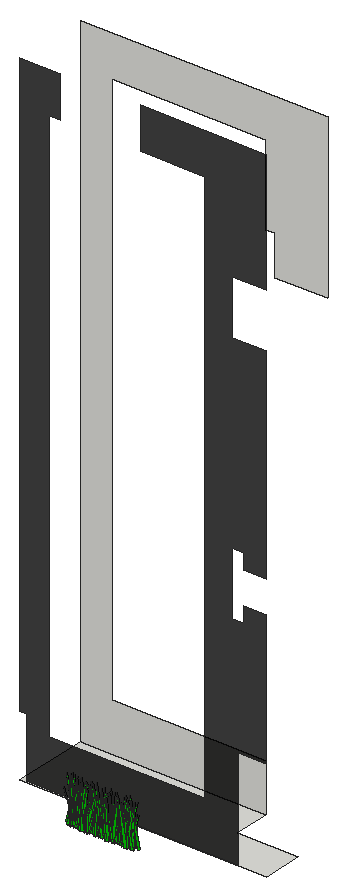
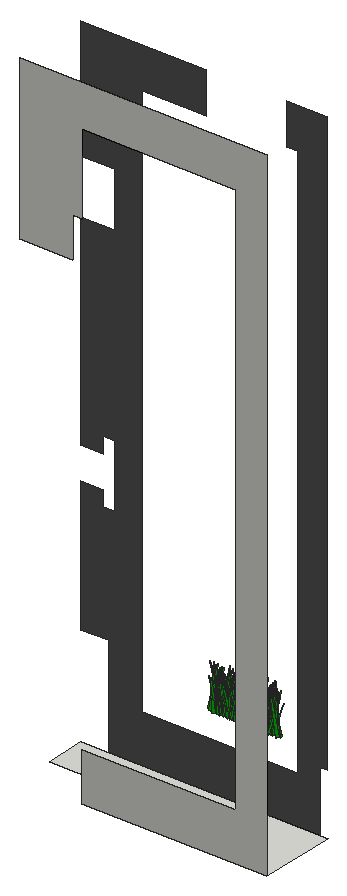
# SketchUp Ruby script. Lengths in inches.
U = 1.inch
M = Sketchup.active_model
def pt(a) = Geom::Point3d.new(a.map { |v| v * U })
def face(e, loops, mat)
  f = e.add_face(loops[0].map { |a| pt(a) })
  loops[1..].each { |l| e.add_face(l.map { |a| pt(a) }).erase! }
  f.material = f.back_material = mat if mat
  f
end
# faces: each face lists its corners as indices into pts; further lists are holes
def faces(e, pts, list, mat = nil) = list.each { |f| face(e, (f[0].is_a?(Array) ? f : [f]).map { |l| l.map { |i| pts[i] } }, mat) }
# xy, xz, yz: faces in a plane at the given z, y or x. An outline is a flat list of corners, or four numbers for a rectangle; further outlines are holes
def ring(l) = l.size == 4 ? [[l[0], l[1]], [l[2], l[1]], [l[2], l[3]], [l[0], l[3]]] : l.each_slice(2).to_a
def flat(e, list, mat, &to3) = list.each { |f| face(e, (f[0].is_a?(Array) ? f : [f]).map { |l| ring(l).map { |u, v| to3.(u, v) } }, mat) }
def xy(e, z, list, mat = nil) = flat(e, list, mat) { |x, y| [x, y, z] }
def xz(e, y, list, mat = nil) = flat(e, list, mat) { |x, z| [x, y, z] }
def yz(e, x, list, mat = nil) = flat(e, list, mat) { |y, z| [x, y, z] }
def lines(e, pts, list) = list.each { |a, b| e.add_line(pt(pts[a]), pt(pts[b])) }
# prism: a flat outline (further loops are holes) pulled along v
def prism(e, loops, v, mat = nil)
  f = face(e, loops, mat); d = Geom::Vector3d.new(v.map { |x| x * U })
  f.pushpull(f.normal.samedirection?(d) ? d.length : -d.length)
end
def box(e, o, s, mat = nil) = prism(e, [[o, [o[0] + s[0], o[1], o[2]], [o[0] + s[0], o[1] + s[1], o[2]], [o[0], o[1] + s[1], o[2]]]], [0, 0, s[2]], mat)
def at(x, y, z, deg = 0) = Geom::Transformation.translation(pt([x, y, z])) * Geom::Transformation.rotation(ORIGIN, Z_AXIS, deg.degrees)
def axes(o, x, y, z) = Geom::Transformation.new([*x, 0, *y, 0, *z, 0, *pt(o).to_a, 1])
def part(name) = M.definitions.add(name)
# library, detail: a bought-in or finely detailed component or shape, given as its bounding box
def library(name, o, s) = part(name).tap { |d| box(d.entities, o, s) }
def detail(e, o, s) = box(e.add_group.entities, o, s)
def put(e, d, t, mat = nil) = e.add_instance(d, t).tap { |i| i.material = mat if mat }
def group(e, t, mat = nil) = e.add_group.tap { |g| g.transformation = t; g.material = mat if mat }.entities
root = M.entities
M.materials.add("[Color G06]").color = [0, 204, 0]
M.materials.add("[Color I07]").color = [0, 0, 0]
M.materials["[Color I07]"].alpha = 0.79
c1 = part("fur_instance\#9")
p = [[0.8125,0,1.79],[0.67,-0.02,1.48],[0,-0.11,0],[0,0.11,0]]
faces(c1.entities,p,[[0,1,2,3]])
xy(root,-6,[[0,50.4375,0,79.8125,71,79.8125,71,65.625,94.55,65.625,94.55,50.4375]])
xz(root,50.4375,[[2.44,-6,84.05,-6,84.05,32.52,94.55,32.52,94.55,84,85.8,84.0625,85.8,78.0625,81.61,78.0625,81.61,102,85.8,102,85.8,96,94.55,96,94.55,174.6875,81.61,174.6875,81.61,195.375,94.55,195.375,94.55,242.375,46.35,242.375,46.35,226.18,71,226.18,71,12.68,11.58,12.68,11.58,226.18,15.47,226.18,15.47,242.375,0,242.375,0,17.375,2.44,17.375]],"[Color I07]")
xz(root,79.8125,[[0,-6,0,242.375,94.55,242.375,94.55,180,74.48,180,74.48,195.375,71,195.375,71,226.18,11.58,226.18,11.58,12.68,71,12.68,71,-6]])
put(root,c1,axes([44.51,23.2,4.28],[-3.54509,0.14274,0.85151],[0.77212,0.47511,-1.96873],[0.88106,0.15798,5.15148]),"[Color G06]")
put(root,c1,axes([45.09,23.48,4.28],[-1.82166,0.34556,1.78414],[2.70884,0.19069,1.93525],[-0.4778,-0.23637,4.16953]),"[Color G06]")
put(root,c1,axes([46.25,23.55,4.28],[-4.84362,0.37826,3.53182],[3.333,0.67983,1.8462],[1.3541,-0.32032,8.08908]),"[Color G06]")
put(root,c1,axes([43.88,23.57,4.28],[-3.95994,-0.13546,0.88932],[-0.84613,0.5507,1.22032],[0.76279,-0.09238,5.97047]),"[Color G06]")
put(root,c1,axes([49.65,23.55,4.28],[5.17923,0.26142,3.18644],[2.36605,-0.73928,-1.62302],[-1.56903,-0.25188,8.07066]),"[Color G06]")
put(root,c1,axes([50.67,23.32,4.28],[-2.69769,0.27399,1.06941],[1.83268,0.38822,-1.0992],[1.007,0.02748,4.86538]),"[Color G06]")
put(root,c1,axes([56.88,23.5625,4.28],[-4.25805,0.04028,1.29058],[0.46192,0.59179,1.28248],[0.78468,-0.12979,6.24834]),"[Color G06]")
put(root,c1,axes([45.7,23.27,4.28],[2.11895,0.70671,1.8047],[4.98939,-0.32759,1.65079],[-1.49964,-0.09135,8.04226]),"[Color G06]")
put(root,c1,axes([62.1,23.4375,4.28],[-1.88004,0.75275,2.43709],[5.58061,0.21393,2.02573],[-0.81003,-0.27325,8.29964]),"[Color G06]")
put(root,c1,axes([51.63,23.65,4.28],[4.44552,0.10549,2.58087],[1.22575,-0.63033,-1.75656],[-1.43239,-0.21201,6.50674]),"[Color G06]")
put(root,c1,axes([60.68,23.37,4.28],[-4.22727,-0.07602,1.84569],[-0.86752,0.5867,-1.66245],[1.03423,0.18142,6.14953]),"[Color G06]")
put(root,c1,axes([56.74,23.71,4.28],[-0.19459,-0.67981,1.29759],[-4.77626,0.05774,1.87526],[1.30687,0.10981,7.04678]),"[Color G06]")
put(root,c1,axes([46.61,23.25,4.28],[-6.08695,0.08552,0.82543],[0.38611,0.80168,-3.18156],[0.72944,0.28931,8.57207]),"[Color G06]")
put(root,c1,axes([40.97,23.76,4.28],[5.65286,-0.0501,2.42135],[0.07547,-0.79345,-2.27951],[-1.65774,-0.20696,8.15299]),"[Color G06]")
put(root,c1,axes([45.35,23.61,4.28],[4.08445,-0.33976,0.05652],[-2.40368,-0.56006,1.2612],[0.40036,0.10372,6.99537]),"[Color G06]")
put(root,c1,axes([54.27,23.35,4.28],[2.99814,0.33718,1.93611],[1.78076,-0.44278,2.69852],[-2.08657,0.1066,5.08498]),"[Color G06]")
put(root,c1,axes([62.9,23.31,4.28],[2.88924,0.4246,0.75633],[2.60876,-0.38757,2.7335],[-1.64986,0.13074,5.64669]),"[Color G06]")
put(root,c1,axes([54.14,23.91,4.28],[3.12472,-0.62007,0.24573],[-4.34541,-0.43125,-1.5795],[-0.9578,-0.06637,7.96762]),"[Color G06]")
put(root,c1,axes([47.5,23.3125,4.28],[-3.39734,0.42812,0.33611],[2.84215,0.45416,-2.28278],[1.1826,0.13839,6.45178]),"[Color G06]")
put(root,c1,axes([62.16,23.56,4.28],[1.75413,0.72883,2.24788],[5.36188,-0.19484,-2.08953],[0.91096,-0.25663,7.97043]),"[Color G06]")
put(root,c1,axes([44.98,23.57,4.28],[2.73301,-0.63153,3.24486],[-5.02072,-0.33463,1.96447],[0.12991,0.35344,7.65778]),"[Color G06]")
put(root,c1,axes([47.04,23.35,4.28],[-3.80873,0.3681,0.6701],[2.34921,0.51156,-2.45531],[1.28475,0.15586,6.47617]),"[Color G06]")
put(root,c1,axes([43.07,23.8,4.28],[1.98494,-0.79883,1.68409],[-5.72424,-0.23362,2.34093],[1.14892,0.21616,8.75366]),"[Color G06]")
put(root,c1,axes([45.58,23.59,4.28],[-1.2576,0.4007,0.15915],[2.65614,0.15567,1.86003],[-1.10158,-0.08211,4.30322]),"[Color G06]")
put(root,c1,axes([52.92,23.53,4.28],[-1.37532,0.6451,0.86713],[4.61456,0.17628,1.28324],[-0.66623,-0.11068,7.09816]),"[Color G06]")
put(root,c1,axes([55.78,23.5,4.28],[-4.40695,-0.23643,2.93875],[-2.38236,0.58297,-2.59258],[1.03211,0.33612,6.56368]),"[Color G06]")
put(root,c1,axes([55.19,23.55,4.28],[0.9786,0.78748,2.4969],[5.61272,-0.19622,2.19507],[-1.78308,-0.18545,8.27993]),"[Color G06]")
put(root,c1,axes([64.37,23.54,4.28],[-0.38469,0.60361,0.86334],[4.16993,0.02675,2.00178],[-1.2972,-0.09301,6.17884]),"[Color G06]")
put(root,c1,axes([41.99,23.87,4.28],[-3.48804,-0.11817,2.16828],[-0.42937,0.51339,1.67127],[1.62435,-0.11805,5.09781]),"[Color G06]")
put(root,c1,axes([52.0625,23.68,4.28],[2.23393,0.42821,3.02957],[3.13811,-0.39438,1.23473],[-1.9212,-0.14628,5.53956]),"[Color G06]")
put(root,c1,axes([55.55,24.03,4.28],[2.10305,-0.67058,1.59322],[-4.42122,-0.32824,-2.83456],[-2.17141,0.01886,7.31451]),"[Color G06]")
put(root,c1,axes([48.33,23.55,4.28],[5.20728,0.24689,0.32404],[1.69027,-0.71279,1.71182],[-0.56976,0.14181,8.03999]),"[Color G06]")
put(root,c1,axes([57.11,24.25,4.28],[-5.38239,-0.42009,0.46162],[-2.5521,0.6765,4.25161],[1.63026,-0.32792,8.17975]),"[Color G06]")
put(root,c1,axes([61.32,23.51,4.28],[-0.30876,0.76243,0.46443],[5.41529,0.04897,-1.19389],[0.81616,-0.03651,8.09724]),"[Color G06]")
put(root,c1,axes([46.4375,23.64,4.28],[3.12548,0.67267,0.38577],[4.72579,-0.41686,-2.02486],[1.00176,-0.13219,8.34865]),"[Color G06]")
put(root,c1,axes([56.5,23.95,4.28],[4.12533,0.2555,0.67281],[1.83219,-0.50648,-3],[0.4503,-0.2799,6.04264]),"[Color G06]")
put(root,c1,axes([46.74,23.92,4.28],[-3.06003,-0.07059,0.14472],[-0.46957,0.41537,1.09426],[0.21238,-0.09863,4.50459]),"[Color G06]")
put(root,c1,axes([55.53,24.21,4.28],[6.01483,-0.23374,0.31839],[-1.46727,-0.77699,-3.60972],[-0.83799,-0.31726,8.60576]),"[Color G06]")
put(root,c1,axes([39.93,23.67,4.28],[2.75325,0.66588,0.22772],[4.68443,-0.37143,-1.74762],[0.939,-0.09946,8.05067]),"[Color G06]")
put(root,c1,axes([47.41,23.89,4.28],[2.57672,-0.41829,1.05478],[-3.02777,-0.31979,1.95383],[0.57331,0.19112,5.57789]),"[Color G06]")
put(root,c1,axes([63.42,24.03,4.28],[4.38595,0.08594,2.1676],[0.96165,-0.6198,-1.52342],[-1.24839,-0.1755,6.44184]),"[Color G06]")
put(root,c1,axes([54.99,24.08,4.28],[-1.28026,-0.58457,0.66085],[-4.17293,0.16664,-1.1253],[-0.59651,0.08891,6.45369]),"[Color G06]")
put(root,c1,axes([64.34,23.76,4.28],[-2.6052,0.64918,1.97946],[4.64475,0.39431,-1.20009],[1.36139,-0.10299,7.88241]),"[Color G06]")
put(root,c1,axes([61.91,23.91,4.28],[2.69159,0.31638,0.03082],[2.17504,-0.35851,-1.53288],[0.64596,-0.11113,5.03305]),"[Color G06]")
put(root,c1,axes([40.33,24.14,4.28],[5.72745,-0.10287,2.95356],[-0.26545,-0.82618,-2.1557],[-2.09263,-0.17675,8.35726]),"[Color G06]")
put(root,c1,axes([49.69,24.2,4.28],[1.41781,-0.56666,0.72438],[-3.7532,-0.20856,-2.33225],[-1.63149,-0.01267,5.9948]),"[Color G06]")
put(root,c1,axes([41.3125,24,4.28],[3.06688,-0.45258,0.09249],[-3.0522,-0.39799,2.35446],[1.10535,0.15676,6.24473]),"[Color G06]")
put(root,c1,axes([42.89,23.9,4.28],[2.5172,0.59368,1.6217],[4.37953,-0.32514,-1.51125],[0.35053,-0.20096,7.23591]),"[Color G06]")
put(root,c1,axes([61.48,24.17,4.28],[3.38185,-0.03705,1.52445],[0.18095,-0.4505,-2.15437],[-1.03838,-0.19917,4.58951]),"[Color G06]")
put(root,c1,axes([42.625,24.0625,4.28],[-4.9972,0.13364,2.38193],[1.22394,0.71608,1.1205],[1.40014,-0.14899,7.52179]),"[Color G06]")
put(root,c1,axes([63.49,24.09,4.28],[-2.77989,0.07928,2.11152],[0.98461,0.40638,1.14286],[1.16178,-0.15471,4.08385]),"[Color G06]")
put(root,c1,axes([48.11,24.16,4.28],[3.30766,-0.41695,1.64743],[-2.87103,-0.48603,-1.25458],[-1.38293,0.01178,6.54484]),"[Color G06]")
put(root,c1,axes([61.75,24.06,4.28],[-2.77391,0.20467,0.40541],[1.46966,0.36059,1.55019],[-0.26061,-0.14501,4.42682]),"[Color G06]")
put(root,c1,axes([44.8,24.05,4.28],[1.74896,-0.40041,0.88785],[-2.85294,-0.21008,1.66982],[0.67752,0.14903,4.73947]),"[Color G06]")
put(root,c1,axes([39.64,24.24,4.28],[5.64974,-0.19428,1.23208],[-1.20485,-0.78336,-1.84886],[-1.08124,-0.14226,8.49812]),"[Color G06]")
put(root,c1,axes([39.85,23.91,4.28],[2.72081,0.15255,0.64251],[0.9646,-0.37616,1.1354],[-0.67168,0.07774,4.23322]),"[Color G06]")
put(root,c1,axes([53.3,23.79,4.28],[2.65671,0.5577,0.40215],[3.92929,-0.37123,1.15715],[-0.79286,0.02899,7.08217]),"[Color G06]")
put(root,c1,axes([54.17,23.875,4.28],[2.43381,0.45044,1.548],[3.02303,-0.36865,1.706],[-1.53902,-0.01179,5.79905]),"[Color G06]")
put(root,c1,axes([51.53,24.07,4.28],[-2.04284,-0.70104,2.83118],[-5.33888,0.23338,-1.96649],[-0.59926,0.31058,7.86838]),"[Color G06]")
put(root,c1,axes([44.5,23.86,4.28],[-4.15417,0.28819,0.00217],[2.04163,0.57233,-1.07178],[0.3207,0.08944,6.85127]),"[Color G06]")
put(root,c1,axes([59.91,24.05,4.28],[-0.13016,0.55284,2.12054],[3.97697,-0.04891,2.01004],[-1.38377,-0.19257,5.57743]),"[Color G06]")
put(root,c1,axes([45.87,24,4.28],[2.55618,0.68675,1.41258],[4.95813,-0.32395,-1.94955],[0.75123,-0.1987,8.06055]),"[Color G06]")
put(root,c1,axes([42.99,24.01,4.28],[-2.53238,0.21747,1.65072],[1.38084,0.38498,-1.09436],[1.32108,0.01447,4.30814]),"[Color G06]")
put(root,c1,axes([58.58,24.27,4.28],[-2.61414,0.0755,2.46332],[1.18253,0.38167,1.45945],[1.26934,-0.20008,3.71343]),"[Color G06]")
put(root,c1,axes([50.57,24.15,4.28],[-1.11696,-0.62876,2.5567],[-4.74363,0.0991,-1.82938],[-0.86932,0.2671,6.69743]),"[Color G06]")
put(root,c1,axes([46.02,24.06,4.28],[-3.04712,0.01766,1.34514],[-0.09356,0.43065,-1.12292],[0.90405,0.10409,4.41759]),"[Color G06]")
put(root,c1,axes([43.17,24.17,4.28],[-3.05812,0.39751,1.18726],[2.94958,0.39655,1.71874],[-0.2395,-0.19202,6.00736]),"[Color G06]")
put(root,c1,axes([56.01,24.375,4.28],[3.28578,-0.24471,0.80487],[-1.53019,-0.45019,-1.76966],[-1.014,-0.11361,5.27863]),"[Color G06]")
put(root,c1,axes([62.73,24.14,4.28],[-0.90376,0.4146,1.13384],[2.85587,0.07332,2.00496],[-1.12218,-0.1473,4.18933]),"[Color G06]")
put(root,c1,axes([48.09,24.21,4.28],[2.40393,0.18991,0.00068],[1.31198,-0.3229,-1.10894],[0.36536,-0.09005,3.97768]),"[Color G06]")
put(root,c1,axes([63.46,24.15,4.28],[-0.9961,0.40079,0.99068],[2.89747,0.11469,1.17759],[-0.55229,-0.12118,4.3912]),"[Color G06]")
put(root,c1,axes([40.58,24.03,4.28],[-0.4466,0.45106,0.24311],[3.15206,0.0658,-1.08915],[0.74447,-0.00799,4.75726]),"[Color G06]")
put(root,c1,axes([42.8125,24.46,4.28],[-4.15504,-0.47948,0.51622],[-3.37474,0.5792,1.12385],[0.74389,-0.05054,7.98189]),"[Color G06]")
put(root,c1,axes([60.5,24,4.28],[1.68813,0.56454,0.88239],[3.84366,-0.24935,1.90061],[-1.40177,-0.00386,6.27413]),"[Color G06]")
put(root,c1,axes([55.37,24.09,4.28],[5.65183,0.07068,2.33159],[0.19207,-0.80363,1.75835],[-1.62902,0.15045,8.29669]),"[Color G06]")
put(root,c1,axes([55.33,24.5,4.28],[0.78581,-0.61938,0.36737],[-4.38723,-0.11366,-1.05136],[-0.73602,0.01622,6.65912]),"[Color G06]")
put(root,c1,axes([47.44,24.31,4.28],[4.43952,0.31201,1.25584],[2.37827,-0.60123,-1.62061],[-0.23735,-0.18841,7.25138]),"[Color G06]")
put(root,c1,axes([51.07,24.5625,4.28],[5.79548,-0.16457,0.568],[-1.02198,-0.77751,-2.58496],[-0.70194,-0.2267,8.45313]),"[Color G06]")
put(root,c1,axes([54.55,24.25,4.28],[-4.30288,0.56119,0.52641],[3.92617,0.56401,2.61482],[-0.95158,-0.21053,8.40825]),"[Color G06]")
put(root,c1,axes([42.59,24.43,4.28],[-5.8982,0.06961,2.998],[0.87333,0.85046,1.56971],[1.87355,-0.1773,8.70644]),"[Color G06]")
put(root,c1,axes([50.58,24.35,4.28],[-4.32865,-0.47958,0.12967],[-3.29266,0.57188,-2.55051],[-0.9971,0.1935,7.85943]),"[Color G06]")
put(root,c1,axes([49.6,24.29,4.28],[1.40688,0.56713,3.43028],[4.09473,-0.31053,2.14631],[-2.24542,-0.21093,6.06326]),"[Color G06]")
put(root,c1,axes([62.31,24.49,4.28],[4.66324,-0.30284,1.8706],[-2.02829,-0.67249,-1.21192],[-1.47273,-0.03273,7.59218]),"[Color G06]")
put(root,c1,axes([51.13,24.25,4.28],[-3.94492,-0.38238,2.12704],[-3.08877,0.48141,-2.85459],[-0.06468,0.33202,6.58863]),"[Color G06]")
put(root,c1,axes([59.15,24.71,4.28],[-4.43637,-0.22327,0.39637],[-1.39977,0.58086,2.59079],[0.82141,-0.21605,6.55575]),"[Color G06]")
put(root,c1,axes([40.41,24.38,4.28],[2.46253,0.44954,0.96413],[3.26416,-0.32089,-1.43547],[0.39239,-0.15177,5.89061]),"[Color G06]")
put(root,c1,axes([61.42,24.5,4.28],[-3.99335,0.20009,0.3539],[1.443,0.53314,1.7444],[-0.18105,-0.16414,6.09734]),"[Color G06]")
put(root,c1,axes([64.03,24.61,4.28],[1.34286,-0.63699,1.91261],[-4.50143,-0.22963,-1.7255],[-1.4971,0.11908,6.90373]),"[Color G06]")
put(root,c1,axes([60.78,24.54,4.28],[5.13234,-0.48599,0.02058],[-3.42829,-0.70337,1.69883],[0.62736,0.13219,9.11511]),"[Color G06]")
put(root,c1,axes([51.63,24.375,4.28],[-0.09018,0.64332,2.03562],[4.69774,-0.02907,1.52017],[-1.03434,-0.18811,6.72676]),"[Color G06]")
put(root,c1,axes([50.46,24.26,4.28],[1.13478,0.78029,1.74265],[5.55676,-0.18944,1.6613],[-1.33917,-0.12486,8.37009]),"[Color G06]")
put(root,c1,axes([53.44,24.5625,4.28],[4.70911,0.00478,0.21852],[0.05766,-0.64816,-1.148],[-0.13866,-0.1073,6.94404]),"[Color G06]")
put(root,c1,axes([57.39,24.51,4.28],[5.02768,0.51942,0.32927],[3.53143,-0.64571,-3.43669],[1.20507,-0.27481,8.69743]),"[Color G06]")
put(root,c1,axes([64.45,24.32,4.28],[-3.45152,0.6757,0.4479],[4.79872,0.46705,1.66213],[-0.73616,-0.12352,8.73477]),"[Color G06]")
put(root,c1,axes([61.73,24.71,4.28],[1.45781,-0.44582,0.06996],[-3.05079,-0.19609,-1.54168],[-0.9572,-0.05401,5.02019]),"[Color G06]")
put(root,c1,axes([39.71,24.29,4.28],[-4.52994,-0.03667,3.35289],[-1.01498,0.65933,-2.23471],[2.01785,0.24932,6.40295]),"[Color G06]")
put(root,c1,axes([63.4,24.45,4.28],[-4.81346,-0.12909,0.94506],[-1.01716,0.66633,-1.11674],[0.4714,0.11962,7.2403]),"[Color G06]")
put(root,c1,axes([53.65,24.42,4.28],[1.4633,0.57673,1.17434],[4.13153,-0.17447,-1.65686],[0.80815,-0.15232,6.34403]),"[Color G06]")
put(root,c1,axes([45.89,24.53,4.28],[-1.79517,0.56547,2.12356],[4.16017,0.175,2.50246],[-1.07512,-0.26701,6.13745]),"[Color G06]")
put(root,c1,axes([55.8,24.62,4.28],[-2.14454,0.26548,1.49941],[2.14441,0.28021,1.15173],[0.18065,-0.1746,4.12834]),"[Color G06]")
put(root,c1,axes([56.74,24.99,4.28],[-1.87106,-0.81207,0.26817],[-5.43972,0.25289,3.19425],[2.08709,-0.06888,8.56579]),"[Color G06]")
put(root,c1,axes([45.31,24.31,4.28],[1.18339,0.78786,0.24697],[5.55454,-0.16645,1.54729],[-1.04702,0.00742,8.48761]),"[Color G06]")
put(root,c1,axes([42.19,24.38,4.28],[5.69454,-0.01159,2.78996],[-0.71037,-0.78565,2.86371],[-1.72828,0.28472,8.01561]),"[Color G06]")
put(root,c1,axes([45.82,24.77,4.28],[1.2642,-0.64821,2.54776],[-4.50234,-0.25257,-2.39162],[-2.0599,0.15424,6.791]),"[Color G06]")
put(root,c1,axes([63.33,24.88,4.28],[-2.9816,-0.4652,0.83091],[-3.18294,0.42091,1.55769],[1.14336,-0.04138,6.50319]),"[Color G06]")
put(root,c1,axes([41.3,24.7,4.28],[-3.9125,0.29195,0.30304],[2.06348,0.52113,1.83533],[-0.4082,-0.16396,6.37312]),"[Color G06]")
put(root,c1,axes([41.5,24.65,4.28],[5.71281,-0.21336,0.73034],[-1.58533,-0.78946,1.20583],[-0.25817,0.12651,8.75652]),"[Color G06]")
put(root,c1,axes([58.75,24.3125,4.28],[-3.07822,0.60283,0.11637],[4.05978,0.40756,-2.65087],[1.48754,0.13514,7.47556]),"[Color G06]")
put(root,c1,axes([39.35,24.9,4.28],[-2.34274,-0.61283,1.79086],[-4.23713,0.36215,1.85487],[1.67231,0.05906,7.20848]),"[Color G06]")
put(root,c1,axes([54.25,24.77,4.28],[-1.81756,-0.64108,3.42773],[-4.68703,0.34583,1.87861],[2.10408,0.2166,7.14573]),"[Color G06]")
put(root,c1,axes([66.05,24.8,4.28],[-1.41834,-0.59176,1.51099],[-4.29946,0.16453,-1.61307],[-0.73842,0.17867,6.48986]),"[Color G06]")
put(root,c1,axes([63.24,24.97,4.28],[3.03856,-0.11775,0.93443],[-0.39946,-0.37621,-2.54456],[-0.97181,-0.21354,3.96761]),"[Color G06]")
put(root,c1,axes([51.95,24.89,4.28],[5.13527,-0.16864,1.27565],[-1.06694,-0.71957,-1.33343],[-1.026,-0.09578,7.77144]),"[Color G06]")
put(root,c1,axes([46.41,24.67,4.28],[5.17083,-0.16862,2.66268],[-1.50867,-0.74483,1.12602],[-1.53626,0.1639,7.8564]),"[Color G06]")
put(root,c1,axes([61.66,24.97,4.28],[-3.28104,-0.36079,0.71699],[-2.44007,0.45717,1.4847],[0.98505,-0.06925,6.06593]),"[Color G06]")
put(root,c1,axes([46.35,24.74,4.28],[4.82748,-0.4122,2.83806],[-3.31173,-0.68412,1.16895],[-1.1731,0.23506,8.37903]),"[Color G06]")
put(root,c1,axes([43.74,24.54,4.28],[-4.23809,0.15017,2.31767],[0.34752,0.58437,-2.93015],[1.85573,0.23353,5.84177]),"[Color G06]")
put(root,c1,axes([58.77,24.73,4.28],[-3.59659,-0.09006,2.21183],[-1.10376,0.50488,-1.64762],[1.17853,0.19802,5.20688]),"[Color G06]")
put(root,c1,axes([58.53,24.71,4.28],[1.58249,0.7468,1.11645],[5.28911,-0.1912,-2.05421],[1.12467,-0.15162,8.0896]),"[Color G06]")
put(root,c1,axes([46.69,25.08,4.28],[-5.78394,0.13338,0.91184],[1.10837,0.75864,2.95697],[0.24208,-0.28673,8.24789]),"[Color G06]")
put(root,c1,axes([43.25,24.72,4.28],[2.91795,0.16125,0.66574],[0.95635,-0.39408,1.60188],[-0.78804,0.11883,4.40909]),"[Color G06]")
put(root,c1,axes([43.34,24.95,4.28],[-2.71546,-0.61692,2.23449],[-4.66889,0.36359,-1.14254],[0.09556,0.23377,7.67369]),"[Color G06]")
put(root,c1,axes([42.74,25.05,4.28],[5.74411,-0.1567,2.3323],[-0.93481,-0.82655,-1.23666],[-1.68051,-0.07583,8.65988]),"[Color G06]")
put(root,c1,axes([58.3125,24.87,4.28],[3.97115,-0.12011,0.19014],[-0.8628,-0.53171,1.6675],[0.11707,0.15573,5.83979]),"[Color G06]")
put(root,c1,axes([43.26,25.07,4.28],[-1.87989,-0.71455,1.70872],[-5.09196,0.20687,-2.57576],[-1.27946,0.22658,7.74036]),"[Color G06]")
put(root,c1,axes([39.15,25.125,4.28],[-0.85405,-0.66897,1.89765],[-4.81658,0.155,1.43479],[1.19487,0.14665,7.14006]),"[Color G06]")
put(root,c1,axes([55.41,24.68,4.28],[-2.56264,0.64357,0.22052],[4.53032,0.35497,-1.40627],[0.89341,0.04602,7.76345]),"[Color G06]")
put(root,c1,axes([59.45,25.04,4.28],[2.78731,-0.41437,0.74392],[-3.00188,-0.37384,1.20345],[0.25784,0.12701,5.96908]),"[Color G06]")
put(root,c1,axes([50.27,24.94,4.28],[-1.1584,0.46676,0.98437],[3.19274,0.11416,2.17406],[-1.20181,-0.14661,4.82682]),"[Color G06]")
put(root,c1,axes([57.3125,24.79,4.28],[0.73187,0.57831,0.53367],[4.06865,-0.11006,1.23747],[-0.87915,-0.02794,6.17123]),"[Color G06]")
put(root,c1,axes([52.66,24.83,4.28],[4.3291,-0.03366,1.95235],[-0.65273,-0.59472,2.05501],[-1.15699,0.20956,6.14573]),"[Color G06]")
put(root,c1,axes([62.56,25.16,4.28],[-1.42056,-0.39619,0.66454],[-2.74324,0.20744,1.10811],[0.86297,0.00724,4.61643]),"[Color G06]")
put(root,c1,axes([62.16,24.94,4.28],[1.84916,0.54995,0.95611],[3.78057,-0.20904,-2.51987],[1.29251,-0.17535,6.00269]),"[Color G06]")
put(root,c1,axes([45.61,25.17,4.28],[3.56317,-0.34704,1.83567],[-2.31811,-0.52542,-1.35979],[-1.526,-0.01219,6.35188]),"[Color G06]")
put(root,c1,axes([56.125,25.02,4.28],[3.93325,0.43328,0.33623],[3.01538,-0.5168,-2.29005],[0.78269,-0.18634,7.13293]),"[Color G06]")
put(root,c1,axes([62.18,24.92,4.28],[-5.45392,0.2052,2.08087],[1.26534,0.7805,-1.43346],[1.58202,0.08315,8.3202]),"[Color G06]")
put(root,c1,axes([51.81,24.97,4.28],[-1.44163,0.76805,1.67507],[5.26461,0.12799,3.3795],[-1.96903,-0.22013,7.8094]),"[Color G06]")
put(root,c1,axes([43.31,25.27,4.28],[1.70389,-0.31321,0.17492],[-2.11063,-0.22974,-1.3307],[-0.77707,-0.06276,3.99793]),"[Color G06]")
put(root,c1,axes([52.47,24.86,4.28],[-0.69322,0.84917,1.20885],[5.99083,0.06833,2.15984],[-1.3594,-0.13189,8.90194]),"[Color G06]")
put(root,c1,axes([51.45,24.96,4.28],[-2.72045,0.3572,1.68043],[2.33113,0.41036,-1.59054],[1.54654,0.0098,5.35343]),"[Color G06]")
put(root,c1,axes([56.16,25.05,4.28],[4.35596,-0.38281,1.37424],[-2.89353,-0.56796,2.31272],[0.09616,0.25064,7.33959]),"[Color G06]")
put(root,c1,axes([53.82,25.08,4.28],[2.13079,0.35803,0.05614],[2.40258,-0.27557,-1.80358],[0.90632,-0.11123,4.64915]),"[Color G06]")
put(root,c1,axes([49.47,24.95,4.28],[-0.97208,0.6492,1.50234],[4.56492,0.16781,-1.73209],[1.35878,-0.09931,6.89389]),"[Color G06]")
put(root,c1,axes([59.74,25.02,4.28],[4.17315,-0.08891,0.69303],[-0.74074,-0.56144,1.68931],[-0.2699,0.16615,6.0791]),"[Color G06]")
put(root,c1,axes([38.12,25.04,4.28],[5.93117,-0.14383,1.01853],[-1.1552,-0.81066,1.87639],[-0.44018,0.18951,8.79977]),"[Color G06]")
put(root,c1,axes([53.4,25.2,4.28],[1.5565,-0.47421,0.79478],[-3.08229,-0.15581,2.80449],[1.53194,0.16832,4.83517]),"[Color G06]")
put(root,c1,axes([42.73,25.33,4.28],[-3.30417,-0.16186,0.86327],[-0.95818,0.45341,1.5733],[0.87336,-0.1149,4.99212]),"[Color G06]")
put(root,c1,axes([62.86,25,4.28],[3.0381,0.08239,1.30201],[0.20945,-0.41096,1.89571],[-1.03158,0.15921,4.21945]),"[Color G06]")
put(root,c1,axes([42.35,25.06,4.28],[-2.83595,0.7432,1.12812],[5.25589,0.35663,2.52434],[-1.16226,-0.20071,8.66277]),"[Color G06]")
put(root,c1,axes([44.43,25.03,4.28],[2.66425,0.3883,2.13061],[2.46983,-0.42135,1.92233],[-1.91991,-0.00319,5.4296]),"[Color G06]")
put(root,c1,axes([62.96,25.02,4.28],[-2.62548,0.60131,0.13674],[4.21035,0.35406,1.71861],[-0.936,-0.09401,7.34711]),"[Color G06]")
put(root,c1,axes([38.9,25.48,4.28],[-1.73651,-0.82671,1.67491],[-5.62772,0.28056,2.87493],[2.1755,0.06589,8.77398]),"[Color G06]")
put(root,c1,axes([63.36,25.37,4.28],[3.86849,0.39281,3.78766],[3.56736,-0.54782,-1.61221],[-1.27742,-0.34027,6.96812]),"[Color G06]")
put(root,c1,axes([46.22,25.41,4.28],[4.20287,-0.30263,1.79696],[-1.9866,-0.60806,-1.38471],[-1.48621,-0.04301,6.93256]),"[Color G06]")
put(root,c1,axes([49.9,25.25,4.28],[3.18507,0.49169,1.50983],[3.66747,-0.42417,-1.4138],[0.05405,-0.19284,6.95942]),"[Color G06]")
put(root,c1,axes([41.92,25.49,4.28],[3.27436,-0.18949,0.38715],[-1.21811,-0.43894,-1.66627],[-0.65559,-0.13083,5.02962]),"[Color G06]")
put(root,c1,axes([44.23,25.2,4.28],[-3.9403,-0.11407,0.71114],[-0.92157,0.52709,-1.69395],[0.21504,0.16877,5.77117]),"[Color G06]")
put(root,c1,axes([49.83,25.36,4.28],[-2.58462,-0.64658,1.83588],[-4.7622,0.32257,-1.92545],[-0.57482,0.23492,7.69679]),"[Color G06]")
put(root,c1,axes([43.79,25.09,4.28],[5.19712,0.25525,1.64586],[1.56241,-0.72965,1.97877],[-1.45678,0.12806,7.99391]),"[Color G06]")
put(root,c1,axes([41.57,25.09,4.28],[1.92477,0.27741,0.02416],[1.76792,-0.23994,1.87642],[-0.91233,0.12029,3.68712]),"[Color G06]")
put(root,c1,axes([59.52,25.36,4.28],[-3.69047,0.24622,1.52658],[1.96524,0.50807,1.19884],[0.54668,-0.16428,5.99582]),"[Color G06]")
put(root,c1,axes([40.85,25.05,4.28],[-4.52428,0.38106,1.2437],[2.43906,0.62845,-2.30036],[1.48699,0.12858,7.55726]),"[Color G06]")
put(root,c1,axes([48.81,25.51,4.28],[-3.72605,-0.17072,0.69572],[-1.06445,0.50874,1.60664],[0.76322,-0.12392,5.63729]),"[Color G06]")
put(root,c1,axes([45.22,25.53,4.28],[-3.83598,-0.1168,2.43875],[-0.22843,0.55379,2.24429],[1.81989,-0.17669,5.42213]),"[Color G06]")
put(root,c1,axes([49.43,25.52,4.28],[3.01583,-0.06059,1.06045],[-0.20022,-0.41396,-1.44492],[-0.80754,-0.12363,4.3186]),"[Color G06]")
put(root,c1,axes([56.5,25,4.28],[3.4467,0.4748,0.45857],[2.86476,-0.43428,3.55605],[-1.86562,0.21031,6.30772]),"[Color G06]")
put(root,c1,axes([54.89,25.51,4.28],[-3.16333,0.05109,0.05375],[0.35511,0.41198,1.69584],[-0.09718,-0.15772,4.44707]),"[Color G06]")
put(root,c1,axes([45.22,25.24,4.28],[-3.65989,-0.0571,0.11637],[-0.4087,0.47284,-2.06205],[-0.08168,0.19236,5.10324]),"[Color G06]")
put(root,c1,axes([50.02,25.26,4.28],[2.71263,0.08809,0.20551],[0.55663,-0.36029,1.32902],[-0.32885,0.11679,3.94486]),"[Color G06]")
put(root,c1,axes([47.64,25.16,4.28],[-4.33807,0.26301,1.45228],[1.52549,0.60098,-2.32448],[1.47466,0.15202,6.67683]),"[Color G06]")
put(root,c1,axes([45.82,25.2,4.28],[-1.01382,0.51068,0.54997],[3.44949,0.15039,-1.83827],[1.28381,-0.00082,5.37357]),"[Color G06]")
put(root,c1,axes([42.625,25.38,4.28],[-2.11506,0.4062,1.01238],[2.98437,0.27913,1.06155],[-0.19468,-0.13414,5.2745]),"[Color G06]")
put(root,c1,axes([61.87,25.72,4.28],[3.32691,-0.56361,0.13572],[-3.9782,-0.45931,-1.28303],[-0.71983,-0.06644,7.71805]),"[Color G06]")
put(root,c1,axes([64.86,25.54,4.28],[1.04893,-0.76962,3.07418],[-5.55445,-0.22618,-2.2712],[-1.95956,0.22914,8.08341]),"[Color G06]")
put(root,c1,axes([43.36,25.38,4.28],[-2.51911,0.34433,0.11574],[2.41142,0.33936,1.26065],[-0.53688,-0.09136,5.11913]),"[Color G06]")
put(root,c1,axes([52.45,25.34,4.28],[1.27564,0.69044,2.62115],[5.1035,-0.22247,1.18374],[-1.24311,-0.20483,7.54948]),"[Color G06]")
put(root,c1,axes([40.02,25.21,4.28],[3.45198,0.63695,2.03513],[4.34387,-0.51691,2.12647],[-1.962,-0.02378,8.28865]),"[Color G06]")
put(root,c1,axes([59,25.36,4.28],[-0.02259,0.80721,3.05508],[5.67667,-0.10578,3.3043],[-2.33726,-0.26471,7.99583]),"[Color G06]")
put(root,c1,axes([52.57,25.66,4.28],[-6.19646,0.03191,0.54307],[0.31811,0.83345,2.48129],[0.28848,-0.23355,8.92903]),"[Color G06]")
put(root,c1,axes([63.66,25.72,4.28],[-0.61428,-0.59182,0.05481],[-4.09129,0.08394,1.69756],[1.12921,-0.01781,6.18033]),"[Color G06]")
put(root,c1,axes([60.08,25.59,4.28],[-5.54411,0.13017,1.83179],[1.16773,0.77144,1.59715],[1.00498,-0.17826,8.24953]),"[Color G06]")
put(root,c1,axes([46.17,25.55,4.28],[3.26404,0.29999,0.64774],[2.13495,-0.40901,-2.27101],[0.50792,-0.20864,5.38321]),"[Color G06]")
put(root,c1,axes([45.67,25.5,4.28],[-3.05236,0.27465,0.22948],[1.92058,0.40331,1.61381],[-0.46278,-0.13771,5.18386]),"[Color G06]")
put(root,c1,axes([55.52,25.66,4.28],[-0.50476,-0.53578,1.22765],[-3.82901,0.09297,1.14434],[0.88089,0.09711,5.67763]),"[Color G06]")
put(root,c1,axes([45.45,25.35,4.28],[4.5692,0.05857,2.95801],[-0.16045,-0.669,2.07541],[-2.01688,0.18592,6.53621]),"[Color G06]")
put(root,c1,axes([62.74,25.59,4.28],[-0.87606,-0.49882,2.45291],[-3.58987,0.19739,1.74717],[1.6133,0.16834,5.21973]),"[Color G06]")
put(root,c1,axes([55.24,25.54,4.28],[5.07822,0.47215,0.00117],[3.26009,-0.68177,-2.46508],[0.91434,-0.19142,8.78272]),"[Color G06]")
put(root,c1,axes([51.33,25.52,4.28],[1.0351,0.47531,1.99055],[3.36999,-0.19905,1.5455],[-1.42668,-0.12532,5.09485]),"[Color G06]")
put(root,c1,axes([42.53,25.65,4.28],[-4.78657,-0.35909,0.10915],[-2.55716,0.65967,-1.18601],[-0.31237,0.10223,8.03643]),"[Color G06]")
put(root,c1,axes([50.43,25.68,4.28],[2.34721,0.28182,0.98626],[2.0462,-0.26226,-2.2691],[0.57697,-0.21637,4.035]),"[Color G06]")
put(root,c1,axes([56.73,25.72,4.28],[-5.28789,0.05779,1.44954],[0.5831,0.73633,1.37926],[0.87886,-0.14083,7.80646]),"[Color G06]")
put(root,c1,axes([54.92,25.37,4.28],[3.76117,0.49142,1.94706],[3.07973,-0.55048,2.67128],[-2.15215,0.07109,7.22534]),"[Color G06]")
put(root,c1,axes([51.17,25.52,4.28],[-2.97668,-0.05987,2.21026],[-0.85637,0.43736,-1.21537],[1.27983,0.15341,4.32747]),"[Color G06]")
put(root,c1,axes([56.97,25.4,4.28],[0.47045,0.72385,0.26289],[4.89128,-0.05346,-2.64262],[1.74699,-0.04525,7.32809]),"[Color G06]")
put(root,c1,axes([51.13,25.71,4.28],[-0.10849,-0.47216,1.754],[-3.30566,-0.05003,-2.00385],[-1.38368,0.15655,4.64974]),"[Color G06]")
put(root,c1,axes([64.28,25.53,4.28],[-5.01838,0.00791,0.94106],[-0.12376,0.6766,-2.12722],[0.61997,0.19906,7.19286]),"[Color G06]")
put(root,c1,axes([39.02,25.57,4.28],[0.25228,0.73323,1.7783],[5.20556,0.01007,-2.12672],[1.40228,-0.16931,7.5749]),"[Color G06]")
put(root,c1,axes([60.92,25.54,4.28],[-0.81682,0.42828,0.3683],[2.93578,0.11897,-1.34864],[0.93539,0.0006,4.55439]),"[Color G06]")
put(root,c1,axes([45.67,25.7,4.28],[-2.96252,0.40592,0.0858],[2.78671,0.39202,1.88139],[-0.84333,-0.13057,5.91549]),"[Color G06]")
put(root,c1,axes([54.24,25.46,4.28],[-5.30707,0.36412,0.73565],[2.4048,0.72338,-2.37811],[1.13025,0.17059,8.51401]),"[Color G06]")
put(root,c1,axes([52.6,25.5,4.28],[-4.08656,0.38896,0.87787],[2.58421,0.56595,-1.9345],[1.20306,0.10555,7.13729]),"[Color G06]")
put(root,c1,axes([51.58,25.69,4.28],[-5.98696,-0.12109,0.2281],[-0.8817,0.8216,-1.58808],[-0.00389,0.14969,8.90103]),"[Color G06]")
put(root,c1,axes([43.6,25.46,4.28],[-4.15955,0.13698,0.92046],[0.51157,0.50387,-3.44987],[1.04045,0.29988,5.37604]),"[Color G06]")
put(root,c1,axes([47.35,25.53,4.28],[1.8085,0.60594,0.22045],[4.13039,-0.24639,2.10973],[-1.35794,0.05756,6.71069]),"[Color G06]")
put(root,c1,axes([57.09,25.72,4.28],[3.3622,0.02398,1.88363],[-0.13072,-0.48753,1.23403],[-1.26525,0.11408,4.87794]),"[Color G06]")
put(root,c1,axes([61.38,25.58,4.28],[5.20692,0.10814,1.91291],[0.17889,-0.68647,3.37028],[-1.48578,0.29632,7.10958]),"[Color G06]")
